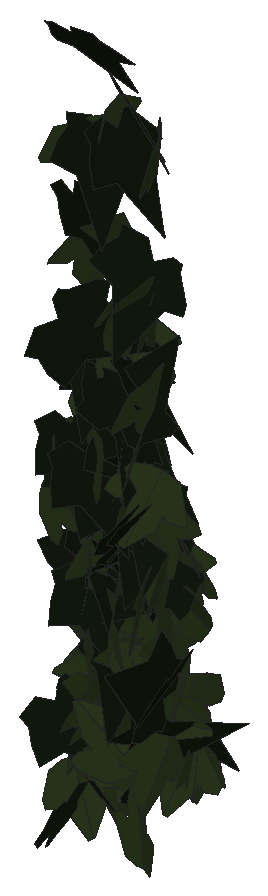
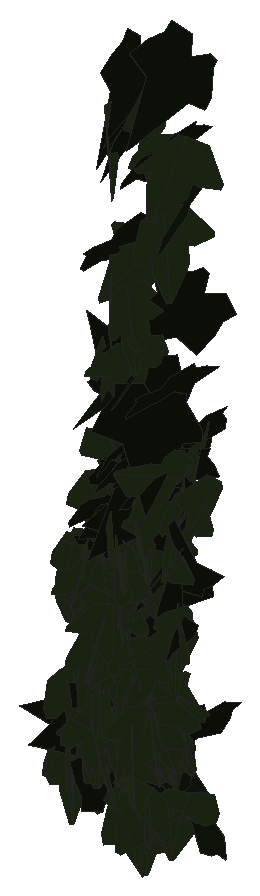
# SketchUp Ruby script. Lengths in inches.
U = 1.inch
M = Sketchup.active_model
def pt(a) = Geom::Point3d.new(a.map { |v| v * U })
def face(e, loops, mat)
  f = e.add_face(loops[0].map { |a| pt(a) })
  loops[1..].each { |l| e.add_face(l.map { |a| pt(a) }).erase! }
  f.material = f.back_material = mat if mat
  f
end
# faces: each face lists its corners as indices into pts; further lists are holes
def faces(e, pts, list, mat = nil) = list.each { |f| face(e, (f[0].is_a?(Array) ? f : [f]).map { |l| l.map { |i| pts[i] } }, mat) }
# xy, xz, yz: faces in a plane at the given z, y or x. An outline is a flat list of corners, or four numbers for a rectangle; further outlines are holes
def ring(l) = l.size == 4 ? [[l[0], l[1]], [l[2], l[1]], [l[2], l[3]], [l[0], l[3]]] : l.each_slice(2).to_a
def flat(e, list, mat, &to3) = list.each { |f| face(e, (f[0].is_a?(Array) ? f : [f]).map { |l| ring(l).map { |u, v| to3.(u, v) } }, mat) }
def xy(e, z, list, mat = nil) = flat(e, list, mat) { |x, y| [x, y, z] }
def xz(e, y, list, mat = nil) = flat(e, list, mat) { |x, z| [x, y, z] }
def yz(e, x, list, mat = nil) = flat(e, list, mat) { |y, z| [x, y, z] }
def lines(e, pts, list) = list.each { |a, b| e.add_line(pt(pts[a]), pt(pts[b])) }
# prism: a flat outline (further loops are holes) pulled along v
def prism(e, loops, v, mat = nil)
  f = face(e, loops, mat); d = Geom::Vector3d.new(v.map { |x| x * U })
  f.pushpull(f.normal.samedirection?(d) ? d.length : -d.length)
end
def box(e, o, s, mat = nil) = prism(e, [[o, [o[0] + s[0], o[1], o[2]], [o[0] + s[0], o[1] + s[1], o[2]], [o[0], o[1] + s[1], o[2]]]], [0, 0, s[2]], mat)
def at(x, y, z, deg = 0) = Geom::Transformation.translation(pt([x, y, z])) * Geom::Transformation.rotation(ORIGIN, Z_AXIS, deg.degrees)
def axes(o, x, y, z) = Geom::Transformation.new([*x, 0, *y, 0, *z, 0, *pt(o).to_a, 1])
def part(name) = M.definitions.add(name)
# library, detail: a bought-in or finely detailed component or shape, given as its bounding box
def library(name, o, s) = part(name).tap { |d| box(d.entities, o, s) }
def detail(e, o, s) = box(e.add_group.entities, o, s)
def put(e, d, t, mat = nil) = e.add_instance(d, t).tap { |i| i.material = mat if mat }
def group(e, t, mat = nil) = e.add_group.tap { |g| g.transformation = t; g.material = mat if mat }.entities
root = M.entities
M.materials.add("efeu1").color = [18, 25, 13]
M.materials.add("efeu2").color = [43, 57, 29]
c1 = part("ivyleaf_10")
p = [[0,0.5,-0.03],[-0.0625,2.02,-0.43],[-0.19,2.01,-0.46],[-0.54,1.05,-0.29],[-0.52,0.625,-0.18],[-0.83,0.76,-0.28],
  [-1.16,0.64,-0.33],[-1.15,0.33,-0.24],[-0.77,-0.39,0.02],[-0.3,-0.51,0.16],[0.04,-0.48,0.23],[-0.02,2.01,-0.4375],
  [-0.06,2.01,-0.43],[0.04,-0.49,0.23],[0.67,-0.49,0.14],[1.38,0.36,-0.2],[1.375,0.51,-0.24],[0.81,0.65,-0.19],
  [0.62,0.59,-0.15],[0.6,1.09,-0.28],[0.5,1.23,-0.31]]
faces(c1.entities,p,[[0,1,2,3,4,5,6,7,8,9,10],[11,12,0,13,14,15,16,17,18,19,20]],"efeu2")
c2 = part("ivyleaf_9")
p = [[1.54,2.16,1.25],[1.36,2.04,1.19],[-0.21,0.99,0.68],[-0.71,1.11,0.82],[-0.85,0.86,0.67],[-0.8,0.17,0.21],
  [-0.9,-0.01,0.1],[-0.67,-0.16,-0.02],[-0.08,-0.08,-0.05],[-0.03,-0.6,-0.4],[0.65,-0.88,-0.66],[0.83,-0.6,-0.49],
  [1.29,-0.42,-0.43],[1.8125,-0.07,-0.26],[1.21,0.44,0.15]]
faces(c2.entities,p,[[0,1,2,3,4,5,6,7,8,9,10,11,12,13,14]],"efeu1")
put(root,c1,axes([525.33,136.5,186.16],[-0.44936,-0.52397,0.23775],[-0.04198,-0.27101,-0.6766],[0.57386,-0.43012,0.13668]))
put(root,c1,axes([525.22,136.72,186.27],[0.63306,0.32594,-0.16511],[-0.17351,-0.0225,-0.70968],[-0.32155,0.65385,0.05789]))
put(root,c1,axes([525.4,136,187.93],[-0.64621,0.29281,0.17903],[-0.21157,-0.03933,-0.69933],[-0.27023,-0.66939,0.1194]))
put(root,c1,axes([525.72,136.9,183.4],[0.17934,0.00919,0.70771],[-0.69365,0.1474,0.17386],[-0.14068,-0.71505,0.04493]))
put(root,c1,axes([525.08,135.89,183.8],[0.44169,0.56045,0.16679],[0.0694,0.1573,-0.71236],[-0.58061,0.44516,0.04174]))
put(root,c1,axes([525.24,134.97,191],[-0.10729,0.60223,0.49338],[-0.08795,0.48548,-0.61171],[-0.77354,-0.13872,0.00112]))
put(root,c1,axes([525.08,136.51,192.125],[0.33094,0.25071,-0.71224],[0.29921,0.67044,0.37503],[0.69326,-0.40904,0.17814]))
put(root,c1,axes([525.71,136.27,186.09],[-0.5393,-0.1143,0.4786],[-0.4581,-0.14255,-0.55026],[0.17961,-0.70681,0.03358]))
put(root,c1,axes([525.31,136.75,186.23],[0.46732,-0.55935,-0.13133],[-0.01401,0.15814,-0.7234],[0.57439,0.45895,0.0892]))
put(root,c1,axes([525.29,135.65,190.92],[-0.025,-0.68682,-0.38033],[0.13051,0.37159,-0.67962],[0.77417,-0.08482,0.10229]))
put(root,c2,axes([525.26,134.87,182.99],[-0.32713,0.74766,-0.00718],[-0.00776,0.00444,0.81608],[0.74766,0.32718,0.00533]))
put(root,c1,axes([525.54,136.5625,185.91],[-0.56358,-0.39166,0.28473],[-0.14061,-0.28572,-0.67133],[0.46335,-0.56308,0.1426]))
put(root,c1,axes([525.41,137.04,184.03],[-0.59021,0.40233,-0.00681],[-0.06842,-0.11225,-0.70213],[-0.39653,-0.57948,0.13128]))
put(root,c1,axes([525.46,136.01,185.79],[0.07409,-0.75275,-0.07547],[-0.01546,0.07431,-0.75634],[0.75636,0.07525,-0.00807]))
put(root,c1,axes([525.16,136,188.11],[0.01245,-0.2504,-0.73782],[0.38297,0.64459,-0.21229],[0.67854,-0.35921,0.13336]))
put(root,c1,axes([525.79,136.97,185.28],[-0.20616,0.11741,0.68981],[-0.57085,0.38766,-0.23659],[-0.40467,-0.60668,-0.01768]))
put(root,c2,axes([525.08,135.27,185.74],[0.2629,-0.48913,-0.52554],[-0.02199,0.55392,-0.52654],[0.7176,0.19617,0.1764]))
put(root,c1,axes([525.3,137.07,184.29],[-0.68189,0.00203,-0.23138],[0.23054,-0.05572,-0.6799],[-0.01982,-0.71792,0.05211]))
put(root,c1,axes([525.29,136.96,186.22],[-0.42965,-0.53371,-0.25998],[0.30808,0.07387,-0.6608],[0.50746,-0.49672,0.18107]))
put(root,c1,axes([525.36,135.125,192.2],[-0.18111,0.74708,-0.10848],[0.0279,-0.10486,-0.76872],[-0.7544,-0.18323,-0.00239]))
put(root,c2,axes([525.79,135.69,189.18],[-0.73764,-0.08579,0.17903],[0.18466,-0.04359,0.73995],[-0.07288,0.7578,0.06283]))
put(root,c2,axes([525.69,136.19,193.56],[0.39185,0.65063,-0.26938],[-0.16334,-0.21589,-0.75904],[-0.68499,0.42368,0.0269]))
put(root,c1,axes([525.61,135.97,185.51],[0.09677,-0.63529,0.37446],[0.04358,-0.37208,-0.64252],[0.73615,0.10554,-0.01119]))
put(root,c2,axes([525.43,136.24,194.13],[-0.16035,-0.75,0.06774],[0.00177,-0.06963,-0.76678],[0.75306,-0.15954,0.01623]))
put(root,c2,axes([525.47,135.33,201.91],[0.76627,0.21565,-0.16634],[-0.18984,0.06679,-0.78793],[-0.19528,0.78127,0.11327]))
put(root,c1,axes([525.8,136.77,183.77],[-0.39593,-0.59563,0.10264],[-0.06396,-0.08072,-0.71517],[0.60101,-0.40097,-0.0085]))
put(root,c1,axes([525.84,135.74,186.14],[-0.71102,-0.21664,0.04594],[-0.0429,-0.01685,-0.74328],[0.21726,-0.7123,0.00361]))
put(root,c1,axes([525.63,135.45,199.54],[-0.61785,-0.4569,-0.25888],[0.2563,0.08653,-0.76442],[0.45835,-0.66428,0.07849]))
put(root,c1,axes([525.65,135.94,190.77],[0.11763,0.65612,0.32799],[-0.02897,0.33608,-0.66191],[-0.73296,0.09201,0.0788]))
put(root,c1,axes([525.69,136.53,187.57],[-0.31372,-0.58889,-0.31315],[0.21296,0.2395,-0.66374],[0.63205,-0.37299,0.06821]))
put(root,c2,axes([525.52,135.18,192.5625],[0.15533,-0.693,-0.30453],[-0.04812,0.30121,-0.70998],[0.75543,0.16168,0.0174]))
put(root,c1,axes([525.8125,136.24,189.89],[-0.63786,-0.39899,-0.13729],[0.1416,0.03201,-0.75088],[0.39748,-0.65168,0.04718]))
put(root,c2,axes([525.83,136.22,187.875],[0.6598,-0.17942,0.43297],[-0.39392,0.1928,0.68018],[-0.25394,-0.76526,0.06985]))
put(root,c2,axes([525.49,136.12,189.53],[0.18091,-0.71439,0.18817],[0.03444,-0.18537,-0.73684],[0.73795,0.18378,-0.01174]))
put(root,c1,axes([526.11,135.87,186.28],[-0.26325,0.3868,0.60638],[-0.39796,0.45955,-0.4659],[-0.59912,-0.4752,0.04303]))
put(root,c1,axes([526.1,134.93,189.42],[0.32482,-0.50816,-0.65821],[-0.25326,0.61262,-0.59794],[0.79204,0.40429,0.07874]))
put(root,c1,axes([525.98,136.41,189.69],[-0.2005,-0.68078,0.27221],[0.03148,-0.28994,-0.70193],[0.73251,-0.17388,0.10467]))
put(root,c1,axes([525.95,136.4,190.82],[0.32368,-0.689,-0.06926],[0.00679,0.0796,-0.7602],[0.69243,0.3213,0.03983]))
put(root,c2,axes([525.52,136.11,189.6875],[0.51231,-0.54222,0.14142],[0.09849,-0.10151,-0.74597],[0.55164,0.52169,0.00184]))
put(root,c2,axes([525.56,135.46,184.27],[0.67559,-0.35581,0.01874],[0.01657,-0.00876,-0.76355],[0.35592,0.67579,-0.00003]))
put(root,c1,axes([525.99,135.68,189.74],[-0.10242,-0.76074,-0.06956],[0.12817,0.05208,-0.75823],[0.75308,-0.11233,0.11958]))
put(root,c2,axes([525.75,135.65,188.82],[-0.02304,-0.67202,-0.39365],[0.02645,0.39292,-0.67232],[0.77838,-0.03325,0.01119]))
put(root,c1,axes([526.06,135.19,192.16],[0.60029,-0.44845,-0.19135],[-0.10151,0.1819,-0.74476],[0.47688,0.60322,0.08233]))
put(root,c2,axes([525.79,135.67,192.01],[-0.20271,-0.62426,-0.40755],[0.17095,0.37217,-0.65509],[0.72565,-0.26206,0.04048]))
put(root,c2,axes([525.64,135.15,198.1],[0.50246,-0.62396,-0.03767],[-0.0315,0.02299,-0.80105],[0.6243,0.50334,-0.0101]))
put(root,c1,axes([526.17,135.22,197.43],[-0.26357,-0.77427,-0.03397],[0.00511,0.03415,-0.81788],[0.775,-0.26355,-0.00616]))
put(root,c1,axes([525.92,135.55,186.88],[-0.40174,0.47041,0.54519],[0.36705,-0.40333,0.61847],[0.61951,0.54402,-0.01289]))
put(root,c1,axes([526.58,135.82,186.92],[-0.36129,0.2033,0.63139],[-0.62446,0.1382,-0.40182],[-0.22368,-0.7142,0.10197]))
put(root,c2,axes([525.81,134.49,195.54],[0.19015,-0.00504,-0.81571],[-0.01969,0.83731,-0.00976],[0.81549,0.02139,0.18997]))
put(root,c1,axes([525.98,136.25,189.83],[-0.49998,0.42483,-0.36369],[0.19566,-0.32413,-0.64761],[-0.5239,-0.52649,0.10522]))
put(root,c1,axes([526.1,136.68,187.88],[0.4868,-0.56554,-0.00913],[0.06103,0.06449,-0.74096],[0.56231,0.4826,0.08831]))
put(root,c1,axes([526.26,136.92,185.96],[0.05679,-0.72834,-0.05716],[0.0065,0.05783,-0.73047],[0.73055,0.0561,0.01095]))
put(root,c2,axes([525.9375,135.63,191.39],[0.67264,0.41599,0.13611],[0.11083,0.07954,-0.79083],[-0.42342,0.68165,0.00921]))
put(root,c1,axes([526.09,136.59,187.1],[-0.39825,0.55492,-0.26846],[0.14204,-0.2284,-0.68284],[-0.59986,-0.4225,0.01654]))
put(root,c1,axes([526.25,136.57,184.78],[0.7594,0.06037,-0.11549],[-0.11572,-0.00152,-0.76176],[-0.05991,0.76813,0.00757]))
put(root,c2,axes([526,135.09,192.07],[0.15269,-0.67184,-0.37989],[-0.03882,0.38008,-0.68777],[0.77083,0.15222,0.04061]))
put(root,c2,axes([526.05,135.53,199.51],[-0.00952,-0.80788,0.00172],[0.00032,-0.00172,-0.80794],[0.80788,-0.00952,0.00034]))
put(root,c2,axes([526.05,135.52,191.3125],[0.2514,-0.55105,-0.46574],[-0.13104,0.45013,-0.60332],[0.70951,0.27839,0.0536]))
put(root,c1,axes([526.35,136.81,186.26],[0.13396,-0.72577,0.02753],[0.00489,-0.02709,-0.73803],[0.72628,0.13405,-0.00011]))
put(root,c1,axes([525.8,135.65,188.05],[0.39194,-0.11506,0.7151],[0.69533,-0.1679,-0.40812],[0.20281,0.798,0.01724]))
put(root,c1,axes([525.86,136.74,189.64],[0.38361,-0.0376,0.63466],[0.63575,0.02761,-0.38264],[-0.00423,0.74107,0.04646]))
put(root,c1,axes([526.3,136.55,189.99],[0.32256,-0.64916,0.20141],[0.16755,-0.14011,-0.71994],[0.65871,0.35352,0.0845]))
put(root,c1,axes([526.38,136.15,189.59],[0.21878,-0.65907,-0.30655],[0.08444,0.34102,-0.6729],[0.72195,0.15983,0.1716]))
put(root,c2,axes([526.35,136.17,191.79],[-0.54492,-0.54449,-0.25806],[0.18227,0.18267,-0.77032],[0.57431,-0.57459,-0.00036]))
put(root,c1,axes([526.48,136.07,195.82],[-0.0392,-0.77444,-0.07693],[0.0006,0.077,-0.77542],[0.77825,-0.03906,-0.00327]))
put(root,c1,axes([526.61,136.02,186.53],[0.25745,-0.39341,-0.56744],[-0.23236,0.52092,-0.46658],[0.65021,0.34193,0.05795]))
put(root,c1,axes([526.54,135.88,187.24],[-0.08423,-0.69939,0.27486],[-0.00667,-0.27587,-0.70402],[0.75144,-0.08085,0.02456]))
put(root,c1,axes([526.58,137,185.81],[-0.62674,-0.36102,0.03365],[-0.02868,-0.01763,-0.72329],[0.36145,-0.6274,0.00096]))
put(root,c1,axes([526.625,135.09,200.26],[-0.13352,0.75234,0.29595],[-0.31168,0.22887,-0.72243],[-0.74596,-0.23029,0.24888]))
put(root,c1,axes([526.35,136.79,188.44],[0.47262,0.56844,0.00239],[0.00186,0.00156,-0.73925],[-0.56844,0.47263,-0.00043]))
put(root,c1,axes([526.6875,135.4,185],[0.34889,0.58122,0.41477],[-0.2278,-0.34691,0.67775],[0.67673,-0.41643,0.01431]))
put(root,c1,axes([526.28,135.73,192.15],[0.51573,-0.44161,0.32341],[0.25841,-0.19529,-0.67873],[0.48254,0.57657,0.01782]))
put(root,c1,axes([526.54,136.36,190.41],[0.16324,-0.74617,0.0146],[0.00791,-0.01322,-0.7638],[0.74627,0.16336,0.0049]))
put(root,c1,axes([526.35,136.05,194.64],[0.29946,0.75244,0.04328],[0.01556,0.04039,-0.80984],[-0.75352,0.29987,0.00048]))
put(root,c2,axes([526.24,136.15,192.14],[0.08218,-0.76174,-0.10428],[-0.00298,0.10455,-0.76611],[0.76884,0.08183,0.00818]))
put(root,c1,axes([526.34,135.51,184.98],[-0.49452,-0.39185,-0.37432],[0.35277,0.15189,-0.62505],[0.41136,-0.60133,0.08604]))
put(root,c2,axes([526.25,135.88,187.12],[0.04795,-0.71629,0.32908],[0.0032,-0.32951,-0.71769],[0.78826,0.04491,-0.0171]))
put(root,c1,axes([526.6875,137.01,185.4],[0.50292,-0.56422,-0.30564],[-0.21773,0.21525,-0.75562],[0.60362,0.54774,-0.0179]))
put(root,c1,axes([526.6,136.82,186.25],[0.1327,-0.72563,-0.02654],[0.00234,0.02741,-0.73763],[0.72611,0.13252,0.00723]))
put(root,c2,axes([526.39,136.37,192.54],[0.00538,-0.7004,0.29604],[-0.00222,-0.29606,-0.70041],[0.76039,0.00409,-0.00414]))
put(root,c1,axes([526.46,136.75,188.6],[0.71981,0.13529,0.10598],[0.09873,0.048,-0.73185],[-0.14067,0.72598,0.02864]))
put(root,c1,axes([526.53,136.97,185.7],[0.61009,0.38909,-0.0028],[-0.00786,0.00711,-0.72353],[-0.38902,0.61006,0.01022]))
put(root,c1,axes([526.68,135.81,187.63],[-0.0163,0.50336,0.57724],[0.0003,0.57738,-0.50347],[-0.76589,-0.01049,-0.01249]))
put(root,c2,axes([526.64,134.97,190.11],[0.26955,0.22076,0.68083],[0.31483,0.61679,-0.32463],[-0.64277,0.39467,0.12651]))
put(root,c2,axes([526.56,136.35,189.96],[-0.12513,-0.67016,0.34329],[0.0985,-0.35958,-0.66605],[0.7465,-0.06489,0.14543]))
put(root,c1,axes([526.86,136.51,188.1],[0.31212,-0.4556,-0.5088],[-0.01846,0.55359,-0.50702],[0.68272,0.22325,0.2189]))
put(root,c2,axes([526.6875,136.51,183.875],[0.27062,0.45231,0.56893],[-0.29667,-0.48547,0.52707],[0.66352,-0.40154,0.00362]))
put(root,c1,axes([526.93,135.57,191.29],[0.04194,-0.65864,-0.47305],[0.04848,0.47487,-0.65688],[0.80946,0.00568,0.06386]))
put(root,c2,axes([526.54,135.86,194.14],[0.59994,-0.47201,-0.18385],[-0.09706,0.17259,-0.75982],[0.49717,0.60328,0.07352]))
put(root,c1,axes([527.05,136.38,189.32],[0.27459,0.6496,-0.24477],[-0.33436,-0.10692,-0.65884],[-0.60836,0.35197,0.25162]))
put(root,c1,axes([526.95,135.58,192.6875],[0.45445,-0.63197,0.01893],[0.01093,-0.01545,-0.77841],[0.63216,0.45458,-0.00015]))
put(root,c1,axes([527.01,135.86,186.37],[0.01528,-0.7265,-0.18855],[0.01753,0.18888,-0.72636],[0.75036,0.01038,0.0208]))
put(root,c2,axes([526.87,134.99,190.34],[0.28978,0.39713,0.59081],[0.22385,0.55469,-0.48265],[-0.67577,0.35404,0.09346]))
put(root,c1,axes([526.99,136.55,187.33],[-0.24758,-0.65102,-0.24879],[0.1221,0.21941,-0.69567],[0.68615,-0.27395,0.03403]))
put(root,c2,axes([526.45,136.91,185.76],[0.02506,-0.00634,-0.81179],[0.67545,0.4507,0.01734],[0.45034,-0.67564,0.01918]))
put(root,c2,axes([526.78,135.27,193.17],[-0.4327,0.04813,0.67201],[0.65803,-0.14123,0.43381],[0.1446,0.78669,0.03677]))
put(root,c2,axes([526.95,136.29,190.97],[-0.1564,-0.75027,0.02733],[0.00538,-0.02903,-0.76632],[0.75075,-0.15609,0.01118]))
put(root,c2,axes([526.84,135.11,200.14],[0.31848,-0.67457,-0.37044],[-0.15121,0.33825,-0.74594],[0.7546,0.35249,0.00687]))
put(root,c2,axes([527.52,136.35,189.46],[-0.75242,-0.00849,0.10189],[-0.10191,0.00091,-0.75246],[0.00829,-0.75928,-0.00204]))
put(root,c1,axes([527.38,136.85,184.6],[-0.6571,-0.14991,0.27901],[-0.19225,-0.32189,-0.62572],[0.25171,-0.63719,0.25045]))
put(root,c1,axes([527.36,137.05,184.68],[-0.68504,0.16311,0.18269],[-0.19303,-0.02557,-0.70096],[-0.15074,-0.70852,0.06735]))
put(root,c1,axes([527.09,136.55,189.23],[0.14594,0.73782,0.07411],[-0.02073,0.07956,-0.75127],[-0.74124,0.14304,0.0356]))
put(root,c1,axes([527.38,136.25,186.05],[-0.58501,-0.39711,0.13249],[-0.09542,-0.09519,-0.70663],[0.40761,-0.59222,0.02474]))
put(root,c2,axes([527.18,134.96,201.08],[0.69529,-0.06271,-0.48765],[-0.47907,0.10352,-0.69638],[0.11056,0.84292,0.04924]))
put(root,c1,axes([527.31,135.62,196.0625],[0.32655,-0.65672,-0.3272],[-0.03464,0.34394,-0.7249],[0.7329,0.30887,0.11152]))
put(root,c1,axes([526.74,135.91,185.83],[0.06479,0.0345,0.76569],[0.62097,0.44807,-0.07273],[-0.44929,0.62426,0.00989]))
put(root,c1,axes([527.18,136.38,189.03],[0.35271,-0.65596,0.04882],[0.17021,0.03751,-0.72573],[0.63537,0.35409,0.16732]))
put(root,c1,axes([527.46,136.76,186.37],[-0.37675,-0.61699,0.15743],[-0.07088,-0.14115,-0.72281],[0.6328,-0.38314,0.01277]))
put(root,c1,axes([527.31,137.05,184.72],[0.26678,-0.66212,-0.10822],[0.04758,0.13484,-0.7077],[0.66922,0.25437,0.09346]))
put(root,c1,axes([527.33,134.56,196.03],[0.21137,0.13712,0.75103],[-0.18175,0.76591,-0.08868],[-0.74149,-0.14865,0.23582]))
put(root,c1,axes([527.35,135.94,185.08],[-0.15811,-0.6558,0.34889],[0.09156,-0.37119,-0.65622],[0.73716,-0.09455,0.15634]))
put(root,c1,axes([527.83,136.41,188.27],[-0.4155,0.1747,-0.59545],[-0.58444,0.13072,0.44617],[0.20859,0.71422,0.06399]))
put(root,c1,axes([527.37,135.65,190.78],[-0.63309,-0.38631,-0.09643],[0.10868,0.00658,-0.73992],[0.38305,-0.64035,0.05057]))
put(root,c1,axes([527.44,136.63,189.64],[-0.56653,0.46554,0.14458],[-0.11526,0.08746,-0.73325],[-0.47365,-0.57811,0.00549]))
put(root,c2,axes([526.81,135.67,185.09],[0.32253,0.05696,0.7663],[0.72765,0.24446,-0.32443],[-0.24696,0.79466,0.04487]))
put(root,c1,axes([527.4,135.37,194.04],[-0.07966,-0.73738,-0.25761],[0.06827,0.25138,-0.74067],[0.77809,-0.09754,0.03862]))
put(root,c1,axes([527.25,135.47,189.35],[0.42261,-0.58527,0.27221],[0.16935,-0.21343,-0.72181],[0.62286,0.45513,0.01156]))
put(root,c1,axes([527.64,134.76,183.37],[-0.09216,0.5831,-0.5662],[-0.239,0.5252,0.57977],[0.77684,0.23075,0.1112]))
put(root,c1,axes([527.4,135.62,199.74],[0.35421,-0.69697,-0.18728],[0.00658,0.21173,-0.77552],[0.72166,0.34016,0.099]))
put(root,c2,axes([527.6,135.77,186.88],[-0.44418,0.56272,-0.38659],[0.24797,-0.29673,-0.71684],[-0.63609,-0.50862,-0.0095]))
put(root,c1,axes([527.45,135.79,189.66],[0.343,-0.67087,-0.24637],[-0.04208,0.25384,-0.7498],[0.71344,0.33751,0.07422]))
put(root,c1,axes([527.47,136.49,189.43],[-0.72615,0.21839,0.02958],[-0.03102,-0.00044,-0.75822],[-0.21819,-0.72675,0.00935]))
put(root,c2,axes([527.3,135.6,196.92],[-0.24668,-0.75446,0.21526],[-0.04,-0.21326,-0.7933],[0.78355,-0.24841,0.02727]))
put(root,c1,axes([527.43,136.42,186.63],[0.46469,-0.57091,-0.03736],[-0.02073,0.0313,-0.73611],[0.57176,0.46514,0.00367]))
put(root,c2,axes([527.45,135.74,186.51],[-0.01299,0.05256,0.8116],[-0.38282,-0.71656,0.04028],[0.71757,-0.38133,0.03618]))
put(root,c1,axes([527.49,135.39,191.77],[0.7105,0.12927,-0.22731],[-0.22417,-0.03775,-0.72215],[-0.13464,0.74502,0.00284]))
